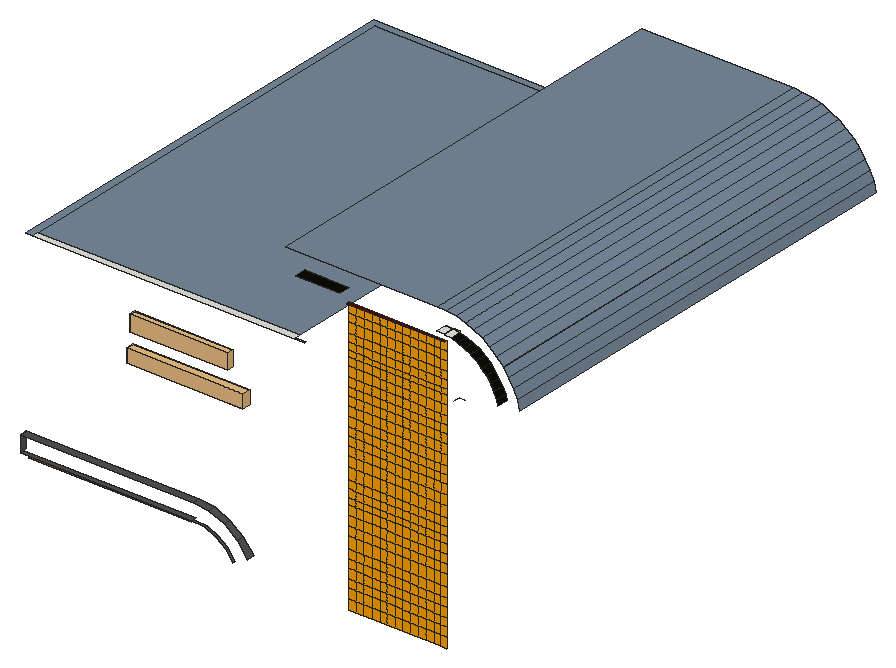
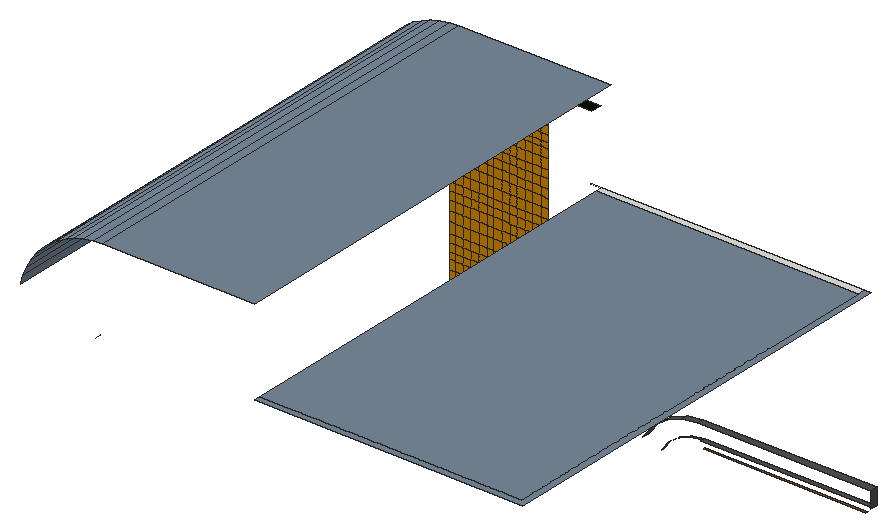
# SketchUp Ruby script. Lengths in inches.
U = 1.inch
M = Sketchup.active_model
def pt(a) = Geom::Point3d.new(a.map { |v| v * U })
def face(e, loops, mat)
  f = e.add_face(loops[0].map { |a| pt(a) })
  loops[1..].each { |l| e.add_face(l.map { |a| pt(a) }).erase! }
  f.material = f.back_material = mat if mat
  f
end
# faces: each face lists its corners as indices into pts; further lists are holes
def faces(e, pts, list, mat = nil) = list.each { |f| face(e, (f[0].is_a?(Array) ? f : [f]).map { |l| l.map { |i| pts[i] } }, mat) }
# xy, xz, yz: faces in a plane at the given z, y or x. An outline is a flat list of corners, or four numbers for a rectangle; further outlines are holes
def ring(l) = l.size == 4 ? [[l[0], l[1]], [l[2], l[1]], [l[2], l[3]], [l[0], l[3]]] : l.each_slice(2).to_a
def flat(e, list, mat, &to3) = list.each { |f| face(e, (f[0].is_a?(Array) ? f : [f]).map { |l| ring(l).map { |u, v| to3.(u, v) } }, mat) }
def xy(e, z, list, mat = nil) = flat(e, list, mat) { |x, y| [x, y, z] }
def xz(e, y, list, mat = nil) = flat(e, list, mat) { |x, z| [x, y, z] }
def yz(e, x, list, mat = nil) = flat(e, list, mat) { |y, z| [x, y, z] }
def lines(e, pts, list) = list.each { |a, b| e.add_line(pt(pts[a]), pt(pts[b])) }
# prism: a flat outline (further loops are holes) pulled along v
def prism(e, loops, v, mat = nil)
  f = face(e, loops, mat); d = Geom::Vector3d.new(v.map { |x| x * U })
  f.pushpull(f.normal.samedirection?(d) ? d.length : -d.length)
end
def box(e, o, s, mat = nil) = prism(e, [[o, [o[0] + s[0], o[1], o[2]], [o[0] + s[0], o[1] + s[1], o[2]], [o[0], o[1] + s[1], o[2]]]], [0, 0, s[2]], mat)
def at(x, y, z, deg = 0) = Geom::Transformation.translation(pt([x, y, z])) * Geom::Transformation.rotation(ORIGIN, Z_AXIS, deg.degrees)
def axes(o, x, y, z) = Geom::Transformation.new([*x, 0, *y, 0, *z, 0, *pt(o).to_a, 1])
def part(name) = M.definitions.add(name)
# library, detail: a bought-in or finely detailed component or shape, given as its bounding box
def library(name, o, s) = part(name).tap { |d| box(d.entities, o, s) }
def detail(e, o, s) = box(e.add_group.entities, o, s)
def put(e, d, t, mat = nil) = e.add_instance(d, t).tap { |i| i.material = mat if mat }
def group(e, t, mat = nil) = e.add_group.tap { |g| g.transformation = t; g.material = mat if mat }.entities
root = M.entities
M.materials.add("[0021_DarkRed]").color = [96, 0, 0]
M.materials.add("[0038_Orange]").color = [255, 165, 0]
M.materials.add("[0059_DarkOliveGreen]").color = [12, 15, 6]
M.materials.add("[0110_LightSlateGray]").color = [119, 136, 153]
M.materials.add("[0135_DarkGray]").color = [81, 81, 81]
M.materials.add("[Wood Cherry Original]").color = [152, 86, 42]
c1 = library("HOLIDAYS",[0.63,0,0],[83.73,10.16,1])
c2 = library("CHOICE",[0.7,0,0],[64.18,10.16,1])
xy(root,385.5625,[[114.44,190.1875,339.27,193.1875]],"[Wood Cherry Original]")
xy(root,391.9375,[[108.0625,183.5625,345.65,190.1875]],"[0135_DarkGray]")
xy(root,415.07,[[108.0625,183.5625,347.17,193.1875]],"[0135_DarkGray]")
xy(root,660,[[117.0625,193.1875,479.14,202.1875],[479.14,193.1875,493.5,194.875]])
xy(root,660,[[108.0625,193.1875,117.0625,193.1875,117.0625,784.1875,479.14,784.1875,479.14,793.1875,108.0625,793.1875],[117.0625,202.1875,479.14,784.1875]],"[0110_LightSlateGray]")
xy(root,739.49,[[563.08,178.1875,698.89,181.1875]],"[0021_DarkRed]")
xy(root,747.32,[[707.96,178.1875,708,193.1875]],"[0059_DarkOliveGreen]")
xy(root,749.49,[[493.5,178.1875,554.01,193.1875]],"[0059_DarkOliveGreen]")
xy(root,780,[[479.14,178.1875,688.91,793.1875]],"[0110_LightSlateGray]")
xz(root,181.1875,[[563.08,358.98,573.89,372.7],[573.89,358.98,584.58,372.7],[584.58,358.98,595.27,372.7],[595.27,358.98,605.96,372.7],[605.96,358.98,616.64,372.7],
  [616.64,358.98,627.33,372.7],[627.33,358.98,638.02,372.7],[638.02,358.98,648.71,372.7],[648.71,358.98,659.39,372.7],[659.39,358.98,670.08,372.7],
  [670.08,358.98,680.77,372.7],[680.77,358.98,691.46,372.7],[691.46,358.98,698.89,372.7],[563.08,372.7,573.89,385.88],[573.89,372.7,584.58,385.88],
  [584.58,372.7,595.27,385.88],[595.27,372.7,605.96,385.88],[605.96,372.7,616.64,385.88],[616.64,372.7,627.33,385.88],[627.33,372.7,638.02,385.88],
  [638.02,372.7,648.71,385.88],[648.71,372.7,659.39,385.88],[659.39,372.7,670.08,385.88],[670.08,372.7,680.77,385.88],[680.77,372.7,691.46,385.88],
  [691.46,372.7,698.89,385.88],[563.08,385.88,573.89,397.18],[573.89,385.88,584.58,397.18],[584.58,385.88,595.27,397.18],[595.27,385.88,605.96,397.18],
  [605.96,385.88,616.64,397.18],[616.64,385.88,627.33,397.18],[627.33,385.88,638.02,397.18],[638.02,385.88,648.71,397.18],[648.71,385.88,659.39,397.18],
  [659.39,385.88,670.08,397.18],[670.08,385.88,680.77,397.18],[680.77,385.88,691.46,397.18],[691.46,385.88,698.89,397.18],[563.08,397.18,573.89,410.44],
  [573.89,397.18,584.58,410.44],[584.58,397.18,595.27,410.44],[595.27,397.18,605.96,410.44],[605.96,397.18,616.64,410.44],[616.64,397.18,627.33,410.44],
  [627.33,397.18,638.02,410.44],[638.02,397.18,648.71,410.44],[648.71,397.18,659.39,410.44],[659.39,397.18,670.08,410.44],[670.08,397.18,680.77,410.44],
  [680.77,397.18,691.46,410.44],[691.46,397.18,698.89,410.44],[563.08,410.44,573.89,421.85],[573.89,410.44,584.58,421.85],[584.58,410.44,595.27,421.85],
  [595.27,410.44,605.96,421.85],[605.96,410.44,616.64,421.85],[616.64,410.44,627.33,421.85],[627.33,410.44,638.02,421.85],[638.02,410.44,648.71,421.85],
  [648.71,410.44,659.39,421.85],[659.39,410.44,670.08,421.85],[670.08,410.44,680.77,421.85],[680.77,410.44,691.46,421.85],[691.46,410.44,698.89,421.85],
  [563.08,421.85,573.89,434.67],[573.89,421.85,584.58,434.67],[584.58,421.85,595.27,434.67],[595.27,421.85,605.96,434.67],[605.96,421.85,616.64,434.67],
  [616.64,421.85,627.33,434.67],[627.33,421.85,638.02,434.67],[638.02,421.85,648.71,434.67],[648.71,421.85,659.39,434.67],[659.39,421.85,670.08,434.67],
  [670.08,421.85,680.77,434.67],[680.77,421.85,691.46,434.67],[691.46,421.85,698.89,434.67],[563.08,434.67,573.89,450.75],[573.89,434.67,584.58,450.75],
  [584.58,434.67,595.27,450.75],[595.27,434.67,605.96,450.75],[605.96,434.67,616.64,450.75],[616.64,434.67,627.33,450.75],[627.33,434.67,638.02,450.75],
  [638.02,434.67,648.71,450.75],[648.71,434.67,659.39,450.75],[659.39,434.67,670.08,450.75],[670.08,434.67,680.77,450.75],[680.77,434.67,691.46,450.75],
  [691.46,434.67,698.89,450.75],[563.08,450.75,573.89,463.5],[573.89,450.75,584.58,463.5],[584.58,450.75,595.27,463.5],[595.27,450.75,605.96,463.5],
  [605.96,450.75,616.64,463.5],[616.64,450.75,627.33,463.5],[627.33,450.75,638.02,463.5],[638.02,450.75,648.71,463.5],[648.71,450.75,659.39,463.5],
  [659.39,450.75,670.08,463.5],[670.08,450.75,680.77,463.5],[680.77,450.75,691.46,463.5],[691.46,450.75,698.89,463.5],[563.08,463.5,573.89,476.16],
  [573.89,463.5,584.58,476.16],[584.58,463.5,595.27,476.16],[595.27,463.5,605.96,476.16],[605.96,463.5,616.64,476.16],[616.64,463.5,627.33,476.16],
  [627.33,463.5,638.02,476.16],[638.02,463.5,648.71,476.16],[648.71,463.5,659.39,476.16],[659.39,463.5,670.08,476.16],[670.08,463.5,680.77,476.16],
  [680.77,463.5,691.46,476.16],[691.46,463.5,698.89,476.16],[563.08,476.16,573.89,488.67],[573.89,476.16,584.58,488.67],[584.58,476.16,595.27,488.67],
  [595.27,476.16,605.96,488.67],[605.96,476.16,616.64,488.67],[616.64,476.16,627.33,488.67],[627.33,476.16,638.02,488.67],[638.02,476.16,648.71,488.67],
  [648.71,476.16,659.39,488.67],[659.39,476.16,670.08,488.67],[670.08,476.16,680.77,488.67],[680.77,476.16,691.46,488.67],[691.46,476.16,698.89,488.67],
  [563.08,488.67,573.89,497.65],[573.89,488.67,584.58,497.65],[584.58,488.67,595.27,497.65],[595.27,488.67,605.96,497.65],[605.96,488.67,616.64,497.65],
  [616.64,488.67,627.33,497.65],[627.33,488.67,638.02,497.65],[638.02,488.67,648.71,497.65],[648.71,488.67,659.39,497.65],[659.39,488.67,670.08,497.65],
  [670.08,488.67,680.77,497.65],[680.77,488.67,691.46,497.65],[691.46,488.67,698.89,497.65],[563.08,497.65,573.89,509.39],[573.89,497.65,584.58,509.39],
  [584.58,497.65,595.27,509.39],[595.27,497.65,605.96,509.39],[605.96,497.65,616.64,509.39],[616.64,497.65,627.33,509.39],[627.33,497.65,638.02,509.39],
  [638.02,497.65,648.71,509.39],[648.71,497.65,659.39,509.39],[659.39,497.65,670.08,509.39],[670.08,497.65,680.77,509.39],[680.77,497.65,691.46,509.39],
  [691.46,497.65,698.89,509.39],[563.08,509.39,573.89,520.18],[573.89,509.39,584.58,520.18],[584.58,509.39,595.27,520.18],[595.27,509.39,605.96,520.18],
  [605.96,509.39,616.64,520.18],[616.64,509.39,627.33,520.18],[627.33,509.39,638.02,520.18],[638.02,509.39,648.71,520.18],[648.71,509.39,659.39,520.18],
  [659.39,509.39,670.08,520.18],[670.08,509.39,680.77,520.18],[680.77,509.39,691.46,520.18],[691.46,509.39,698.89,520.18],[563.08,520.18,573.89,535.7],
  [573.89,520.18,584.58,535.7],[584.58,520.18,595.27,535.7],[595.27,520.18,605.96,535.7],[605.96,520.18,616.64,535.7],[616.64,520.18,627.33,535.7],
  [627.33,520.18,638.02,535.7],[638.02,520.18,648.71,535.7],[648.71,520.18,659.39,535.7],[659.39,520.18,670.08,535.7],[670.08,520.18,680.77,535.7],
  [680.77,520.18,691.46,535.7],[691.46,520.18,698.89,535.7],[563.08,535.7,573.89,549.18],[573.89,535.7,584.58,549.18],[584.58,535.7,595.27,549.18],
  [595.27,535.7,605.96,549.18],[605.96,535.7,616.64,549.18],[616.64,535.7,627.33,549.18],[627.33,535.7,638.02,549.18],[638.02,535.7,648.71,549.18],
  [648.71,535.7,659.39,549.18],[659.39,535.7,670.08,549.18],[670.08,535.7,680.77,549.18],[680.77,535.7,691.46,549.18],[691.46,535.7,698.89,549.18],
  [563.08,549.18,573.89,562.01],[573.89,549.18,584.58,562.01],[584.58,549.18,595.27,562.01],[595.27,549.18,605.96,562.01],[605.96,549.18,616.64,562.01],
  [616.64,549.18,627.33,562.01],[627.33,549.18,638.02,562.01],[638.02,549.18,648.71,562.01],[648.71,549.18,659.39,562.01],[659.39,549.18,670.08,562.01],
  [670.08,549.18,680.77,562.01],[680.77,549.18,691.46,562.01],[691.46,549.18,698.89,562.01],[563.08,562.01,573.89,573.85],[573.89,562.01,584.58,573.85],
  [584.58,562.01,595.27,573.85],[595.27,562.01,605.96,573.85],[605.96,562.01,616.64,573.85],[616.64,562.01,627.33,573.85],[627.33,562.01,638.02,573.85],
  [638.02,562.01,648.71,573.85],[648.71,562.01,659.39,573.85],[659.39,562.01,670.08,573.85],[670.08,562.01,680.77,573.85],[680.77,562.01,691.46,573.85],
  [691.46,562.01,698.89,573.85],[563.08,573.85,573.89,585.16],[573.89,573.85,584.58,585.16],[584.58,573.85,595.27,585.16],[595.27,573.85,605.96,585.16],
  [605.96,573.85,616.64,585.16],[616.64,573.85,627.33,585.16],[627.33,573.85,638.02,585.16],[638.02,573.85,648.71,585.16],[648.71,573.85,659.39,585.16],
  [659.39,573.85,670.08,585.16],[670.08,573.85,680.77,585.16],[680.77,573.85,691.46,585.16],[691.46,573.85,698.89,585.16],[563.08,585.16,573.89,598.53],
  [573.89,585.16,584.58,598.53],[584.58,585.16,595.27,598.53],[595.27,585.16,605.96,598.53],[605.96,585.16,616.64,598.53],[616.64,585.16,627.33,598.53],
  [627.33,585.16,638.02,598.53],[638.02,585.16,648.71,598.53],[648.71,585.16,659.39,598.53],[659.39,585.16,670.08,598.53],[670.08,585.16,680.77,598.53],
  [680.77,585.16,691.46,598.53],[691.46,585.16,698.89,598.53],[563.08,598.53,573.89,611.7],[573.89,598.53,584.58,611.7],[584.58,598.53,595.27,611.7],
  [595.27,598.53,605.96,611.7],[605.96,598.53,616.64,611.7],[616.64,598.53,627.33,611.7],[627.33,598.53,638.02,611.7],[638.02,598.53,648.71,611.7],
  [648.71,598.53,659.39,611.7],[659.39,598.53,670.08,611.7],[670.08,598.53,680.77,611.7],[680.77,598.53,691.46,611.7],[691.46,598.53,698.89,611.7],
  [563.08,611.7,573.89,623.97],[573.89,611.7,584.58,623.97],[584.58,611.7,595.27,623.97],[595.27,611.7,605.96,623.97],[605.96,611.7,616.64,623.97],
  [616.64,611.7,627.33,623.97],[627.33,611.7,638.02,623.97],[638.02,611.7,648.71,623.97],[648.71,611.7,659.39,623.97],[659.39,611.7,670.08,623.97],
  [670.08,611.7,680.77,623.97],[680.77,611.7,691.46,623.97],[691.46,611.7,698.89,623.97],[563.08,623.97,573.89,635.4],[573.89,623.97,584.58,635.4],
  [584.58,623.97,595.27,635.4],[595.27,623.97,605.96,635.4],[605.96,623.97,616.64,635.4],[616.64,623.97,627.33,635.4],[627.33,623.97,638.02,635.4],
  [638.02,623.97,648.71,635.4],[648.71,623.97,659.39,635.4],[659.39,623.97,670.08,635.4],[670.08,623.97,680.77,635.4],[680.77,623.97,691.46,635.4],
  [691.46,623.97,698.89,635.4],[563.08,635.4,573.89,647.11],[573.89,635.4,584.58,647.11],[584.58,635.4,595.27,647.11],[595.27,635.4,605.96,647.11],
  [605.96,635.4,616.64,647.11],[616.64,635.4,627.33,647.11],[627.33,635.4,638.02,647.11],[638.02,635.4,648.71,647.11],[648.71,635.4,659.39,647.11],
  [659.39,635.4,670.08,647.11],[670.08,635.4,680.77,647.11],[680.77,635.4,691.46,647.11],[691.46,635.4,698.89,647.11],[563.08,647.11,573.89,660.47],
  [573.89,647.11,584.58,660.47],[584.58,647.11,595.27,660.47],[595.27,647.11,605.96,660.47],[605.96,647.11,616.64,660.47],[616.64,647.11,627.33,660.47],
  [627.33,647.11,638.02,660.47],[638.02,647.11,648.71,660.47],[648.71,647.11,659.39,660.47],[659.39,647.11,670.08,660.47],[670.08,647.11,680.77,660.47],
  [680.77,647.11,691.46,660.47],[691.46,647.11,698.89,660.47],[563.08,660.47,573.89,672.46],[573.89,660.47,584.58,672.46],[584.58,660.47,595.27,672.46],
  [595.27,660.47,605.96,672.46],[605.96,660.47,616.64,672.46],[616.64,660.47,627.33,672.46],[627.33,660.47,638.02,672.46],[638.02,660.47,648.71,672.46],
  [648.71,660.47,659.39,672.46],[659.39,660.47,670.08,672.46],[670.08,660.47,680.77,672.46],[680.77,660.47,691.46,672.46],[691.46,660.47,698.89,672.46],
  [563.08,672.46,573.89,680.25],[573.89,672.46,584.58,680.25],[584.58,672.46,595.27,680.25],[595.27,672.46,605.96,680.25],[605.96,672.46,616.64,680.25],
  [616.64,672.46,627.33,680.25],[627.33,672.46,638.02,680.25],[638.02,672.46,648.71,680.25],[648.71,672.46,659.39,680.25],[659.39,672.46,670.08,680.25],
  [670.08,672.46,680.77,680.25],[680.77,672.46,691.46,680.25],[691.46,672.46,698.89,680.25],[563.08,680.25,573.89,690.86],[573.89,680.25,584.58,690.86],
  [584.58,680.25,595.27,690.86],[595.27,680.25,605.96,690.86],[605.96,680.25,616.64,690.86],[616.64,680.25,627.33,690.86],[627.33,680.25,638.02,690.86],
  [638.02,680.25,648.71,690.86],[648.71,680.25,659.39,690.86],[659.39,680.25,670.08,690.86],[670.08,680.25,680.77,690.86],[680.77,680.25,691.46,690.86],
  [691.46,680.25,698.89,690.86],[563.08,690.86,573.89,701.83],[573.89,690.86,584.58,701.83],[584.58,690.86,595.27,701.83],[595.27,690.86,605.96,701.83],
  [605.96,690.86,616.64,701.83],[616.64,690.86,627.33,701.83],[627.33,690.86,638.02,701.83],[638.02,690.86,648.71,701.83],[648.71,690.86,659.39,701.83],
  [659.39,690.86,670.08,701.83],[670.08,690.86,680.77,701.83],[680.77,690.86,691.46,701.83],[691.46,690.86,698.89,701.83],[563.08,701.83,573.89,715.24],
  [573.89,701.83,584.58,715.24],[584.58,701.83,595.27,715.24],[595.27,701.83,605.96,715.24],[605.96,701.83,616.64,715.24],[616.64,701.83,627.33,715.24],
  [627.33,701.83,638.02,715.24],[638.02,701.83,648.71,715.24],[648.71,701.83,659.39,715.24],[659.39,701.83,670.08,715.24],[670.08,701.83,680.77,715.24],
  [680.77,701.83,691.46,715.24],[691.46,701.83,698.89,715.24],[563.08,715.24,573.89,726.98],[573.89,715.24,584.58,726.98],[584.58,715.24,595.27,726.98],
  [595.27,715.24,605.96,726.98],[605.96,715.24,616.64,726.98],[616.64,715.24,627.33,726.98],[627.33,715.24,638.02,726.98],[638.02,715.24,648.71,726.98],
  [648.71,715.24,659.39,726.98],[659.39,715.24,670.08,726.98],[670.08,715.24,680.77,726.98],[680.77,715.24,691.46,726.98],[691.46,715.24,698.89,726.98],
  [563.08,726.98,573.89,739.49],[573.89,726.98,584.58,739.49],[584.58,726.98,595.27,739.49],[595.27,726.98,605.96,739.49],[605.96,726.98,616.64,739.49],
  [616.64,726.98,627.33,739.49],[627.33,726.98,638.02,739.49],[638.02,726.98,648.71,739.49],[648.71,726.98,659.39,739.49],[659.39,726.98,670.08,739.49],
  [670.08,726.98,680.77,739.49],[680.77,726.98,691.46,739.49],[691.46,726.98,698.89,739.49]],"[0038_Orange]")
xz(root,193.1875,[[707.96,747.32,707.96,749.49,698.89,749.49,698.89,748.85],[698.89,748.85,698.89,749.49,688.0625,749.49,698.51,748.91]])
yz(root,108.0625,[[183.5625,391.9375,183.5625,415.07,193.1875,415.07,193.1875,392.57,190.1875,391.9375]],"[0135_DarkGray]")
p = [[391.83,183.5625,372.81],[391.83,186.75,372.81],[402.21,186.75,359.28],[402.21,183.5625,359.28],[422.42,193.1875,370.95],[408.33,193.1875,389.31],
  [408.33,183.5625,389.31],[422.42,183.5625,370.95],[378.31,183.5625,383.1875],[378.31,186.75,383.1875],[362.55,183.5625,389.71],[362.55,186.75,389.71],
  [389.97,193.1875,403.39],[389.97,183.5625,403.39],[345.65,183.5625,391.9375],[345.65,186.75,391.9375],[368.59,193.1875,412.25],[368.59,183.5625,412.25],
  [347.17,193.1875,415.07],[347.17,183.5625,415.07],[770.39,193.1875,692.5],[772.36,193.1875,686.03],[772.36,178.1875,686.03],[770.39,178.1875,692.5],
  [799.09,793.1875,703.01],[799.09,178.1875,703.01],[802.875,178.1875,690.57],[802.875,793.1875,690.57],[766.59,193.1875,701.34],[766.59,178.1875,701.34],
  [761.83,193.1875,709.7],[761.83,178.1875,709.7],[793.95,793.1875,714.96],[793.95,178.1875,714.96],[756.18,193.1875,717.48],[756.18,178.1875,717.48],
  [787.52,793.1875,726.26],[787.52,178.1875,726.26],[749.7,193.1875,724.59],[749.7,178.1875,724.59],[742.48,193.1875,730.93],[742.48,178.1875,730.93],
  [780.13,793.1875,736.43],[780.13,178.1875,736.43],[734.59,193.1875,736.44],[734.59,178.1875,736.44],[726.15,193.1875,741.04],[734.21,178.1875,736.65],
  [726.15,178.1875,741.04],[779.87,793.1875,736.78],[779.87,178.1875,736.78],[771.11,793.1875,746.39],[771.11,178.1875,746.39],[717.25,193.1875,744.68],
  [717.25,178.1875,744.68],[708,193.1875,747.32],[708,178.1875,747.32],[761.34,793.1875,754.97],[761.34,178.1875,754.97],[698.89,193.1875,748.85],
  [707.96,193.1875,747.32],[707.96,178.1875,747.32],[698.89,178.1875,748.85],[698.51,193.1875,748.91],[698.51,178.1875,748.91],[688.0625,193.1875,749.49],
  [688.0625,178.1875,749.49],[750.68,793.1875,762.42],[750.68,178.1875,762.42],[739.26,793.1875,768.65],[739.26,178.1875,768.65],[727.23,793.1875,773.57],
  [727.23,178.1875,773.57],[714.72,793.1875,777.125],[714.72,178.1875,777.125],[701.89,793.1875,779.28],[701.89,178.1875,779.28],[688.91,793.1875,780],
  [688.91,178.1875,780],[699.0625,202.1875,660],[699.0625,193.1875,660],[708.0625,202.1875,660],[699.0625,784.1875,660],[699.0625,793.1875,660],
  [734.21,181.1875,739.49],[734.21,181.1875,736.65]]
faces(root,p,[[0,1,2,3],[4,5,6,7],[8,9,1,0],[10,11,9,8],[5,12,13,6],[14,15,11,10],[12,16,17,13],[16,18,19,17]],"[0135_DarkGray]")
faces(root,p,[[20,21,22,23],[28,20,23,29],[30,28,29,31],[34,30,31,35],[38,34,35,39],[40,38,39,41],[44,40,41,45],[46,44,45,47,48],
  [53,46,48,54],[55,53,54,56]],"[0059_DarkOliveGreen]")
faces(root,p,[[24,25,26,27],[32,33,25,24],[36,37,33,32],[42,43,37,36],[49,50,43,42],[51,52,50,49],[57,58,52,51],[67,68,58,57],
  [69,70,68,67],[71,72,70,69],[73,74,72,71],[75,76,74,73],[77,78,76,75]],"[0110_LightSlateGray]")
faces(root,p,[[59,60,61,62],[63,59,62,64],[65,63,64,66]])
lines(root,p,[[79,80],[79,81],[82,83],[84,85],[85,47]])
put(root,c1,axes([254.62,193.1875,556.05],[1.92287,0,0],[0,0,1.83131],[0,-10.98546,0]))
put(root,c2,axes([256.72,193.1875,594.52],[2.12,0,0],[0,0,2.12],[0,-8.48,0]))
